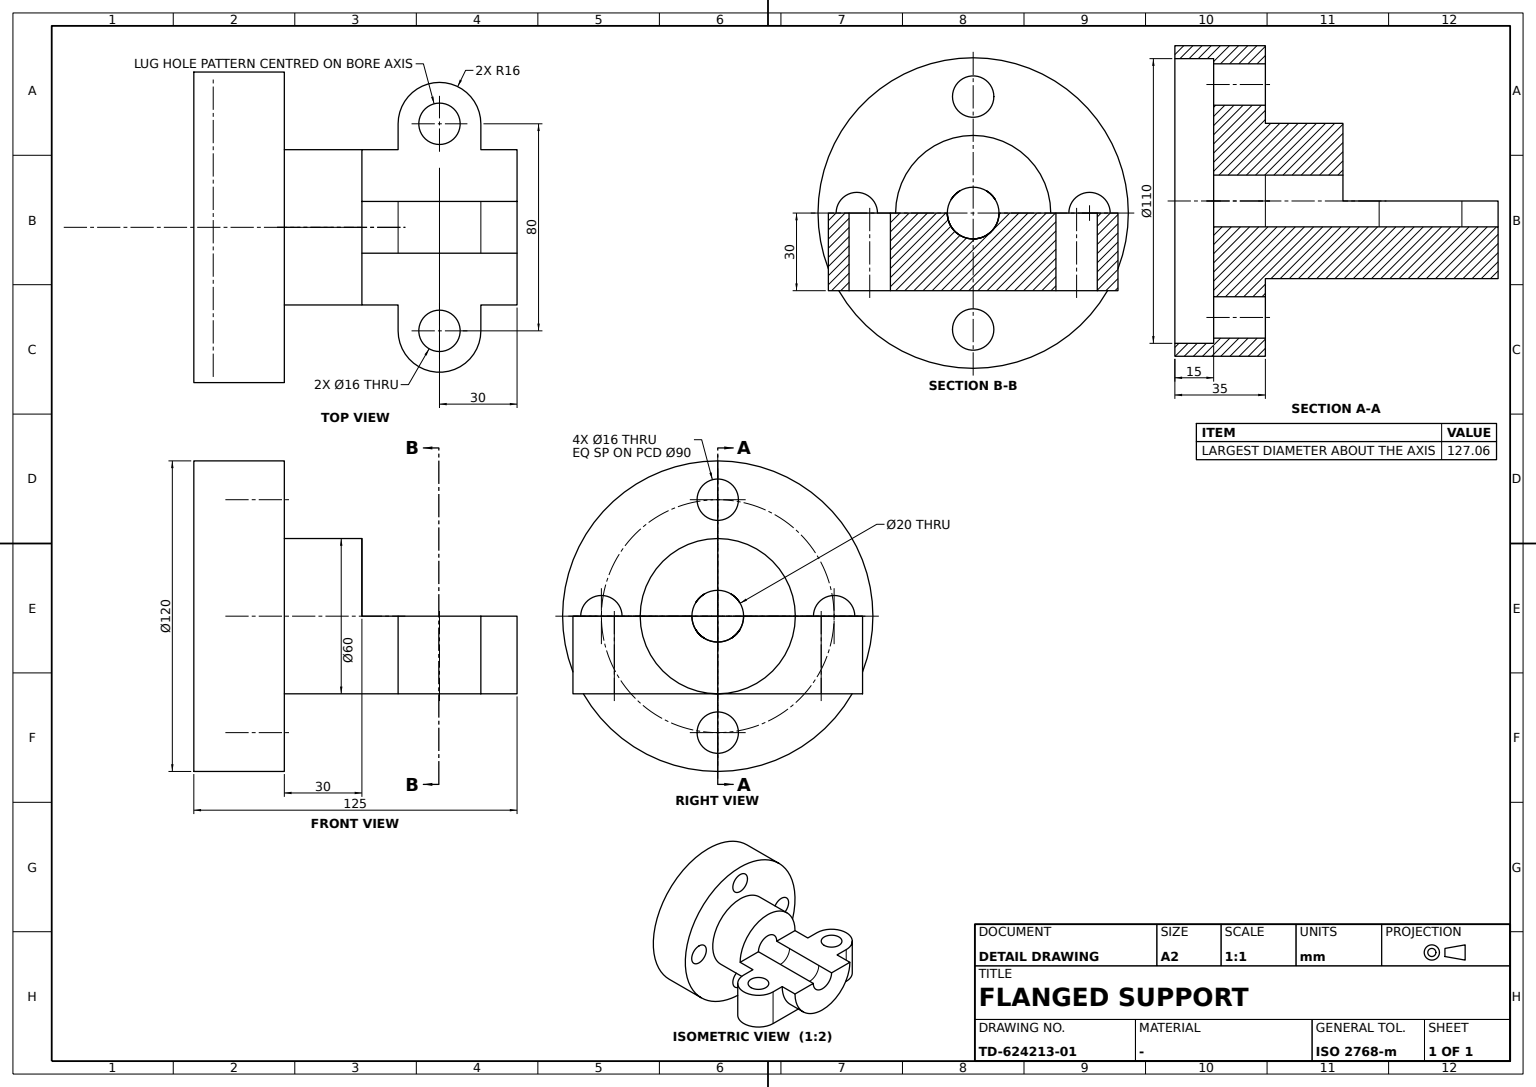
ISO-10303-21;
HEADER;
FILE_DESCRIPTION((''),'2;1');
FILE_NAME('','',(''),(''),'','','');
FILE_SCHEMA(('AUTOMOTIVE_DESIGN'));
ENDSEC;
DATA;
#1=APPLICATION_CONTEXT('');
#2=PRODUCT_CONTEXT('',#1,'mechanical');
#3=PRODUCT('','','',(#2));
#4=PRODUCT_DEFINITION_FORMATION('','',#3);
#5=PRODUCT_DEFINITION_CONTEXT('',#1,'design');
#6=PRODUCT_DEFINITION('','',#4,#5);
#7=PRODUCT_DEFINITION_SHAPE('','',#6);
#8=(LENGTH_UNIT()NAMED_UNIT(*)SI_UNIT(.MILLI.,.METRE.));
#9=(NAMED_UNIT(*)PLANE_ANGLE_UNIT()SI_UNIT($,.RADIAN.));
#10=(NAMED_UNIT(*)SI_UNIT($,.STERADIAN.)SOLID_ANGLE_UNIT());
#11=UNCERTAINTY_MEASURE_WITH_UNIT(LENGTH_MEASURE(1.E-05),#8,'distance_accuracy_value','');
#12=(GEOMETRIC_REPRESENTATION_CONTEXT(3)GLOBAL_UNCERTAINTY_ASSIGNED_CONTEXT((#11))GLOBAL_UNIT_ASSIGNED_CONTEXT((#8,#9,#10))REPRESENTATION_CONTEXT('',''));
#13=CARTESIAN_POINT('',(30.,0.,35.));
#14=VERTEX_POINT('',#13);
#15=CARTESIAN_POINT('',(-30.,0.,35.));
#16=VERTEX_POINT('',#15);
#17=CARTESIAN_POINT('',(0.,0.,35.));
#18=DIRECTION('',(0.,0.,1.));
#19=DIRECTION('',(1.,0.,0.));
#20=AXIS2_PLACEMENT_3D('',#17,#18,#19);
#21=CIRCLE('',#20,30.);
#22=EDGE_CURVE('',#14,#16,#21,.T.);
#23=ORIENTED_EDGE('',*,*,#22,.F.);
#24=EDGE_CURVE('',#16,#14,#21,.T.);
#25=ORIENTED_EDGE('',*,*,#24,.F.);
#26=EDGE_LOOP('',(#23,#25));
#27=FACE_BOUND('',#26,.T.);
#28=CARTESIAN_POINT('',(-8.,45.,35.));
#29=VERTEX_POINT('',#28);
#30=CARTESIAN_POINT('',(8.,45.,35.));
#31=VERTEX_POINT('',#30);
#32=CARTESIAN_POINT('',(0.,45.,35.));
#33=AXIS2_PLACEMENT_3D('',#32,#18,#19);
#34=CIRCLE('',#33,8.);
#35=EDGE_CURVE('',#29,#31,#34,.T.);
#36=ORIENTED_EDGE('',*,*,#35,.F.);
#37=EDGE_CURVE('',#31,#29,#34,.T.);
#38=ORIENTED_EDGE('',*,*,#37,.F.);
#39=EDGE_LOOP('',(#36,#38));
#40=FACE_BOUND('',#39,.T.);
#41=CARTESIAN_POINT('',(-45.,8.,35.));
#42=VERTEX_POINT('',#41);
#43=CARTESIAN_POINT('',(-45.,-8.,35.));
#44=VERTEX_POINT('',#43);
#45=CARTESIAN_POINT('',(-45.,0.,35.));
#46=DIRECTION('',(0.,1.,0.));
#47=AXIS2_PLACEMENT_3D('',#45,#18,#46);
#48=CIRCLE('',#47,8.);
#49=EDGE_CURVE('',#42,#44,#48,.T.);
#50=ORIENTED_EDGE('',*,*,#49,.F.);
#51=EDGE_CURVE('',#44,#42,#48,.T.);
#52=ORIENTED_EDGE('',*,*,#51,.F.);
#53=EDGE_LOOP('',(#50,#52));
#54=FACE_BOUND('',#53,.T.);
#55=CARTESIAN_POINT('',(45.,8.,35.));
#56=VERTEX_POINT('',#55);
#57=CARTESIAN_POINT('',(45.,-8.,35.));
#58=VERTEX_POINT('',#57);
#59=CARTESIAN_POINT('',(45.,0.,35.));
#60=DIRECTION('',(0.,-1.,0.));
#61=AXIS2_PLACEMENT_3D('',#59,#18,#60);
#62=CIRCLE('',#61,8.);
#63=EDGE_CURVE('',#56,#58,#62,.T.);
#64=ORIENTED_EDGE('',*,*,#63,.F.);
#65=EDGE_CURVE('',#58,#56,#62,.T.);
#66=ORIENTED_EDGE('',*,*,#65,.F.);
#67=EDGE_LOOP('',(#64,#66));
#68=FACE_BOUND('',#67,.T.);
#69=CARTESIAN_POINT('',(-8.,-45.,35.));
#70=VERTEX_POINT('',#69);
#71=CARTESIAN_POINT('',(8.,-45.,35.));
#72=VERTEX_POINT('',#71);
#73=CARTESIAN_POINT('',(0.,-45.,35.));
#74=DIRECTION('',(-1.,0.,0.));
#75=AXIS2_PLACEMENT_3D('',#73,#18,#74);
#76=CIRCLE('',#75,8.);
#77=EDGE_CURVE('',#70,#72,#76,.T.);
#78=ORIENTED_EDGE('',*,*,#77,.F.);
#79=EDGE_CURVE('',#72,#70,#76,.T.);
#80=ORIENTED_EDGE('',*,*,#79,.F.);
#81=EDGE_LOOP('',(#78,#80));
#82=FACE_BOUND('',#81,.T.);
#83=CARTESIAN_POINT('',(60.,0.,35.));
#84=VERTEX_POINT('',#83);
#85=CARTESIAN_POINT('',(-60.,0.,35.));
#86=VERTEX_POINT('',#85);
#87=CIRCLE('',#20,60.);
#88=EDGE_CURVE('',#84,#86,#87,.T.);
#89=ORIENTED_EDGE('',*,*,#88,.T.);
#90=EDGE_CURVE('',#86,#84,#87,.T.);
#91=ORIENTED_EDGE('',*,*,#90,.T.);
#92=EDGE_LOOP('',(#89,#91));
#93=FACE_OUTER_BOUND('',#92,.T.);
#94=PLANE('',#20);
#95=ADVANCED_FACE('',(#27,#40,#54,#68,#82,#93),#94,.T.);
#96=CARTESIAN_POINT('',(60.,0.,0.));
#97=VERTEX_POINT('',#96);
#98=CARTESIAN_POINT('',(60.,0.,17.5));
#99=VECTOR('',#18,1000.);
#100=LINE('',#98,#99);
#101=EDGE_CURVE('',#97,#84,#100,.T.);
#102=ORIENTED_EDGE('',*,*,#101,.F.);
#103=CARTESIAN_POINT('',(-60.,0.,0.));
#104=VERTEX_POINT('',#103);
#105=CARTESIAN_POINT('',(0.,0.,0.));
#106=AXIS2_PLACEMENT_3D('',#105,#18,#19);
#107=CIRCLE('',#106,60.);
#108=EDGE_CURVE('',#97,#104,#107,.T.);
#109=ORIENTED_EDGE('',*,*,#108,.T.);
#110=CARTESIAN_POINT('',(-60.,0.,17.5));
#111=LINE('',#110,#99);
#112=EDGE_CURVE('',#104,#86,#111,.T.);
#113=ORIENTED_EDGE('',*,*,#112,.T.);
#114=ORIENTED_EDGE('',*,*,#88,.F.);
#115=EDGE_LOOP('',(#102,#109,#113,#114));
#116=FACE_OUTER_BOUND('',#115,.T.);
#117=CARTESIAN_POINT('',(0.,0.,17.5));
#118=DIRECTION('',(0.,0.,-1.));
#119=AXIS2_PLACEMENT_3D('',#117,#118,#19);
#120=CYLINDRICAL_SURFACE('',#119,60.);
#121=ADVANCED_FACE('',(#116),#120,.T.);
#122=CARTESIAN_POINT('',(0.,30.,111.));
#123=VERTEX_POINT('',#122);
#124=CARTESIAN_POINT('',(30.,0.,111.));
#125=VERTEX_POINT('',#124);
#126=CARTESIAN_POINT('',(0.,0.,111.));
#127=AXIS2_PLACEMENT_3D('',#126,#118,#46);
#128=CIRCLE('',#127,30.);
#129=EDGE_CURVE('',#123,#125,#128,.T.);
#130=ORIENTED_EDGE('',*,*,#129,.T.);
#131=CARTESIAN_POINT('',(30.,40.,111.));
#132=VERTEX_POINT('',#131);
#133=CARTESIAN_POINT('',(30.,20.,111.));
#134=VECTOR('',#60,1000.);
#135=LINE('',#133,#134);
#136=EDGE_CURVE('',#132,#125,#135,.T.);
#137=ORIENTED_EDGE('',*,*,#136,.F.);
#138=CARTESIAN_POINT('',(0.,40.,111.));
#139=VERTEX_POINT('',#138);
#140=CARTESIAN_POINT('',(15.,40.,111.));
#141=VECTOR('',#19,1000.);
#142=LINE('',#140,#141);
#143=EDGE_CURVE('',#139,#132,#142,.T.);
#144=ORIENTED_EDGE('',*,*,#143,.F.);
#145=CARTESIAN_POINT('',(0.,35.,111.));
#146=LINE('',#145,#134);
#147=EDGE_CURVE('',#139,#123,#146,.T.);
#148=ORIENTED_EDGE('',*,*,#147,.T.);
#149=EDGE_LOOP('',(#130,#137,#144,#148));
#150=FACE_OUTER_BOUND('',#149,.T.);
#151=CARTESIAN_POINT('',(0.,-40.,111.));
#152=AXIS2_PLACEMENT_3D('',#151,#118,#46);
#153=PLANE('',#152);
#154=ADVANCED_FACE('',(#150),#153,.F.);
#155=CARTESIAN_POINT('',(0.,-48.,95.));
#156=VERTEX_POINT('',#155);
#157=CARTESIAN_POINT('',(30.,-48.,95.));
#158=VERTEX_POINT('',#157);
#159=CARTESIAN_POINT('',(15.,-48.,95.));
#160=LINE('',#159,#141);
#161=EDGE_CURVE('',#156,#158,#160,.T.);
#162=ORIENTED_EDGE('',*,*,#161,.T.);
#163=CARTESIAN_POINT('',(30.,-32.,95.));
#164=VERTEX_POINT('',#163);
#165=CARTESIAN_POINT('',(30.,-40.,95.));
#166=AXIS2_PLACEMENT_3D('',#165,#19,#46);
#167=CIRCLE('',#166,8.);
#168=EDGE_CURVE('',#158,#164,#167,.T.);
#169=ORIENTED_EDGE('',*,*,#168,.T.);
#170=CARTESIAN_POINT('',(0.,-32.,95.));
#171=VERTEX_POINT('',#170);
#172=CARTESIAN_POINT('',(15.,-32.,95.));
#173=LINE('',#172,#141);
#174=EDGE_CURVE('',#171,#164,#173,.T.);
#175=ORIENTED_EDGE('',*,*,#174,.F.);
#176=CARTESIAN_POINT('',(0.,-40.,95.));
#177=AXIS2_PLACEMENT_3D('',#176,#19,#46);
#178=CIRCLE('',#177,8.);
#179=EDGE_CURVE('',#156,#171,#178,.T.);
#180=ORIENTED_EDGE('',*,*,#179,.F.);
#181=EDGE_LOOP('',(#162,#169,#175,#180));
#182=FACE_OUTER_BOUND('',#181,.T.);
#183=CARTESIAN_POINT('',(15.,-40.,95.));
#184=AXIS2_PLACEMENT_3D('',#183,#74,#46);
#185=CYLINDRICAL_SURFACE('',#184,8.);
#186=ADVANCED_FACE('',(#182),#185,.F.);
#187=CARTESIAN_POINT('',(0.,32.,95.));
#188=VERTEX_POINT('',#187);
#189=CARTESIAN_POINT('',(0.,48.,95.));
#190=VERTEX_POINT('',#189);
#191=CARTESIAN_POINT('',(0.,40.,95.));
#192=AXIS2_PLACEMENT_3D('',#191,#19,#46);
#193=CIRCLE('',#192,8.);
#194=EDGE_CURVE('',#188,#190,#193,.T.);
#195=ORIENTED_EDGE('',*,*,#194,.F.);
#196=CARTESIAN_POINT('',(30.,32.,95.));
#197=VERTEX_POINT('',#196);
#198=CARTESIAN_POINT('',(15.,32.,95.));
#199=LINE('',#198,#141);
#200=EDGE_CURVE('',#188,#197,#199,.T.);
#201=ORIENTED_EDGE('',*,*,#200,.T.);
#202=CARTESIAN_POINT('',(30.,48.,95.));
#203=VERTEX_POINT('',#202);
#204=CARTESIAN_POINT('',(30.,40.,95.));
#205=AXIS2_PLACEMENT_3D('',#204,#19,#46);
#206=CIRCLE('',#205,8.);
#207=EDGE_CURVE('',#197,#203,#206,.T.);
#208=ORIENTED_EDGE('',*,*,#207,.T.);
#209=CARTESIAN_POINT('',(15.,48.,95.));
#210=LINE('',#209,#141);
#211=EDGE_CURVE('',#190,#203,#210,.T.);
#212=ORIENTED_EDGE('',*,*,#211,.F.);
#213=EDGE_LOOP('',(#195,#201,#208,#212));
#214=FACE_OUTER_BOUND('',#213,.T.);
#215=CARTESIAN_POINT('',(15.,40.,95.));
#216=AXIS2_PLACEMENT_3D('',#215,#74,#46);
#217=CYLINDRICAL_SURFACE('',#216,8.);
#218=ADVANCED_FACE('',(#214),#217,.F.);
#219=VERTEX_POINT('',#151);
#220=CARTESIAN_POINT('',(30.,-40.,111.));
#221=VERTEX_POINT('',#220);
#222=CARTESIAN_POINT('',(15.,-40.,111.));
#223=LINE('',#222,#141);
#224=EDGE_CURVE('',#219,#221,#223,.T.);
#225=ORIENTED_EDGE('',*,*,#224,.F.);
#226=CARTESIAN_POINT('',(0.,-40.,79.));
#227=VERTEX_POINT('',#226);
#228=CIRCLE('',#177,16.);
#229=EDGE_CURVE('',#219,#227,#228,.T.);
#230=ORIENTED_EDGE('',*,*,#229,.T.);
#231=CARTESIAN_POINT('',(30.,-40.,79.));
#232=VERTEX_POINT('',#231);
#233=CARTESIAN_POINT('',(15.,-40.,79.));
#234=LINE('',#233,#141);
#235=EDGE_CURVE('',#227,#232,#234,.T.);
#236=ORIENTED_EDGE('',*,*,#235,.T.);
#237=CIRCLE('',#166,16.);
#238=EDGE_CURVE('',#221,#232,#237,.T.);
#239=ORIENTED_EDGE('',*,*,#238,.F.);
#240=EDGE_LOOP('',(#225,#230,#236,#239));
#241=FACE_OUTER_BOUND('',#240,.T.);
#242=CYLINDRICAL_SURFACE('',#184,16.);
#243=ADVANCED_FACE('',(#241),#242,.T.);
#244=CARTESIAN_POINT('',(-10.,0.,65.));
#245=VERTEX_POINT('',#244);
#246=CARTESIAN_POINT('',(0.,-10.,65.));
#247=VERTEX_POINT('',#246);
#248=CARTESIAN_POINT('',(0.,0.,65.));
#249=AXIS2_PLACEMENT_3D('',#248,#18,#19);
#250=CIRCLE('',#249,10.);
#251=EDGE_CURVE('',#245,#247,#250,.T.);
#252=ORIENTED_EDGE('',*,*,#251,.T.);
#253=CARTESIAN_POINT('',(0.,-10.,79.));
#254=VERTEX_POINT('',#253);
#255=CARTESIAN_POINT('',(0.,-10.,72.));
#256=LINE('',#255,#99);
#257=EDGE_CURVE('',#247,#254,#256,.T.);
#258=ORIENTED_EDGE('',*,*,#257,.T.);
#259=CARTESIAN_POINT('',(10.,0.,79.));
#260=VERTEX_POINT('',#259);
#261=CARTESIAN_POINT('',(1.308997,-10.,79.));
#262=CARTESIAN_POINT('',(2.617479,-9.739727,79.));
#263=CARTESIAN_POINT('',(5.03619,-8.737864,79.));
#264=CARTESIAN_POINT('',(6.145467,-7.996668,79.));
#265=CARTESIAN_POINT('',(7.996668,-6.145467,79.));
#266=CARTESIAN_POINT('',(8.737864,-5.03619,79.));
#267=CARTESIAN_POINT('',(9.739727,-2.617479,79.));
#268=CARTESIAN_POINT('',(10.,-1.308997,79.));
#269=B_SPLINE_CURVE_WITH_KNOTS('',3,(#253,#261,#262,#263,#264,#265,#266,#267,#268,#259),.UNSPECIFIED.,.F.,.F.,(4,2,2,2,4),(0.,0.25,0.5,0.75,1.),.UNSPECIFIED.);
#270=EDGE_CURVE('',#254,#260,#269,.T.);
#271=ORIENTED_EDGE('',*,*,#270,.T.);
#272=CARTESIAN_POINT('',(10.,0.,35.));
#273=VERTEX_POINT('',#272);
#274=CARTESIAN_POINT('',(10.,0.,62.5));
#275=LINE('',#274,#99);
#276=EDGE_CURVE('',#273,#260,#275,.T.);
#277=ORIENTED_EDGE('',*,*,#276,.F.);
#278=CARTESIAN_POINT('',(0.,-10.,35.));
#279=VERTEX_POINT('',#278);
#280=CARTESIAN_POINT('',(3.141593,-10.,35.));
#281=CARTESIAN_POINT('',(6.286116,-8.76985,35.));
#282=CARTESIAN_POINT('',(8.76985,-6.286116,35.));
#283=CARTESIAN_POINT('',(10.,-3.141593,35.));
#284=B_SPLINE_CURVE_WITH_KNOTS('',5,(#278,#280,#281,#282,#283,#272),.UNSPECIFIED.,.F.,.F.,(6,6),(0.,1.),.UNSPECIFIED.);
#285=EDGE_CURVE('',#279,#273,#284,.T.);
#286=ORIENTED_EDGE('',*,*,#285,.F.);
#287=CARTESIAN_POINT('',(-10.,0.,35.));
#288=VERTEX_POINT('',#287);
#289=CARTESIAN_POINT('',(-10.,-3.141593,35.));
#290=CARTESIAN_POINT('',(-8.76985,-6.286116,35.));
#291=CARTESIAN_POINT('',(-6.286116,-8.76985,35.));
#292=CARTESIAN_POINT('',(-3.141593,-10.,35.));
#293=B_SPLINE_CURVE_WITH_KNOTS('',5,(#287,#289,#290,#291,#292,#278),.UNSPECIFIED.,.F.,.F.,(6,6),(0.,1.),.UNSPECIFIED.);
#294=EDGE_CURVE('',#288,#279,#293,.T.);
#295=ORIENTED_EDGE('',*,*,#294,.F.);
#296=CARTESIAN_POINT('',(-10.,0.,62.5));
#297=LINE('',#296,#99);
#298=EDGE_CURVE('',#288,#245,#297,.T.);
#299=ORIENTED_EDGE('',*,*,#298,.T.);
#300=EDGE_LOOP('',(#252,#258,#271,#277,#286,#295,#299));
#301=FACE_OUTER_BOUND('',#300,.T.);
#302=CARTESIAN_POINT('',(0.,0.,62.5));
#303=AXIS2_PLACEMENT_3D('',#302,#118,#19);
#304=CYLINDRICAL_SURFACE('',#303,10.);
#305=ADVANCED_FACE('',(#301),#304,.F.);
#306=CARTESIAN_POINT('',(-45.,8.,15.));
#307=VERTEX_POINT('',#306);
#308=CARTESIAN_POINT('',(-45.,8.,16.84));
#309=VECTOR('',#118,1000.);
#310=LINE('',#308,#309);
#311=EDGE_CURVE('',#42,#307,#310,.T.);
#312=ORIENTED_EDGE('',*,*,#311,.T.);
#313=CARTESIAN_POINT('',(-45.,-8.,15.));
#314=VERTEX_POINT('',#313);
#315=CARTESIAN_POINT('',(-45.,0.,15.));
#316=AXIS2_PLACEMENT_3D('',#315,#118,#19);
#317=CIRCLE('',#316,8.);
#318=EDGE_CURVE('',#307,#314,#317,.T.);
#319=ORIENTED_EDGE('',*,*,#318,.T.);
#320=CARTESIAN_POINT('',(-45.,-8.,16.84));
#321=LINE('',#320,#309);
#322=EDGE_CURVE('',#44,#314,#321,.T.);
#323=ORIENTED_EDGE('',*,*,#322,.F.);
#324=ORIENTED_EDGE('',*,*,#51,.T.);
#325=EDGE_LOOP('',(#312,#319,#323,#324));
#326=FACE_OUTER_BOUND('',#325,.T.);
#327=CARTESIAN_POINT('',(-45.,0.,16.84));
#328=AXIS2_PLACEMENT_3D('',#327,#118,#46);
#329=CYLINDRICAL_SURFACE('',#328,8.);
#330=ADVANCED_FACE('',(#326),#329,.F.);
#331=CARTESIAN_POINT('',(0.,-10.,125.));
#332=VERTEX_POINT('',#331);
#333=CARTESIAN_POINT('',(0.,-10.,111.));
#334=VERTEX_POINT('',#333);
#335=CARTESIAN_POINT('',(0.,-10.,118.));
#336=LINE('',#335,#309);
#337=EDGE_CURVE('',#332,#334,#336,.T.);
#338=ORIENTED_EDGE('',*,*,#337,.F.);
#339=CARTESIAN_POINT('',(10.,0.,125.));
#340=VERTEX_POINT('',#339);
#341=CARTESIAN_POINT('',(0.,0.,125.));
#342=AXIS2_PLACEMENT_3D('',#341,#18,#19);
#343=CIRCLE('',#342,10.);
#344=EDGE_CURVE('',#332,#340,#343,.T.);
#345=ORIENTED_EDGE('',*,*,#344,.T.);
#346=CARTESIAN_POINT('',(10.,0.,111.));
#347=VERTEX_POINT('',#346);
#348=EDGE_CURVE('',#347,#340,#275,.T.);
#349=ORIENTED_EDGE('',*,*,#348,.F.);
#350=CARTESIAN_POINT('',(3.141593,-10.,111.));
#351=CARTESIAN_POINT('',(6.286116,-8.76985,111.));
#352=CARTESIAN_POINT('',(8.76985,-6.286116,111.));
#353=CARTESIAN_POINT('',(10.,-3.141593,111.));
#354=B_SPLINE_CURVE_WITH_KNOTS('',5,(#333,#350,#351,#352,#353,#346),.UNSPECIFIED.,.F.,.F.,(6,6),(0.,1.),.UNSPECIFIED.);
#355=EDGE_CURVE('',#334,#347,#354,.T.);
#356=ORIENTED_EDGE('',*,*,#355,.F.);
#357=EDGE_LOOP('',(#338,#345,#349,#356));
#358=FACE_OUTER_BOUND('',#357,.T.);
#359=ADVANCED_FACE('',(#358),#304,.F.);
#360=CARTESIAN_POINT('',(0.,-30.,79.));
#361=VERTEX_POINT('',#360);
#362=CARTESIAN_POINT('',(0.,-30.,65.));
#363=VERTEX_POINT('',#362);
#364=CARTESIAN_POINT('',(0.,-30.,62.5));
#365=LINE('',#364,#309);
#366=EDGE_CURVE('',#361,#363,#365,.T.);
#367=ORIENTED_EDGE('',*,*,#366,.T.);
#368=CARTESIAN_POINT('',(-30.,0.,65.));
#369=VERTEX_POINT('',#368);
#370=CIRCLE('',#249,30.);
#371=EDGE_CURVE('',#369,#363,#370,.T.);
#372=ORIENTED_EDGE('',*,*,#371,.F.);
#373=CARTESIAN_POINT('',(-30.,0.,62.5));
#374=LINE('',#373,#99);
#375=EDGE_CURVE('',#16,#369,#374,.T.);
#376=ORIENTED_EDGE('',*,*,#375,.F.);
#377=ORIENTED_EDGE('',*,*,#24,.T.);
#378=CARTESIAN_POINT('',(30.,0.,79.));
#379=VERTEX_POINT('',#378);
#380=CARTESIAN_POINT('',(30.,0.,62.5));
#381=LINE('',#380,#99);
#382=EDGE_CURVE('',#14,#379,#381,.T.);
#383=ORIENTED_EDGE('',*,*,#382,.T.);
#384=CARTESIAN_POINT('',(0.,0.,79.));
#385=AXIS2_PLACEMENT_3D('',#384,#18,#60);
#386=CIRCLE('',#385,30.);
#387=EDGE_CURVE('',#361,#379,#386,.T.);
#388=ORIENTED_EDGE('',*,*,#387,.F.);
#389=EDGE_LOOP('',(#367,#372,#376,#377,#383,#388));
#390=FACE_OUTER_BOUND('',#389,.T.);
#391=CYLINDRICAL_SURFACE('',#303,30.);
#392=ADVANCED_FACE('',(#390),#391,.T.);
#393=ORIENTED_EDGE('',*,*,#194,.T.);
#394=EDGE_CURVE('',#190,#188,#193,.T.);
#395=ORIENTED_EDGE('',*,*,#394,.T.);
#396=EDGE_LOOP('',(#393,#395));
#397=FACE_BOUND('',#396,.T.);
#398=CARTESIAN_POINT('',(0.,10.,125.));
#399=VERTEX_POINT('',#398);
#400=CARTESIAN_POINT('',(0.,30.,125.));
#401=VERTEX_POINT('',#400);
#402=CARTESIAN_POINT('',(0.,20.,125.));
#403=VECTOR('',#46,1000.);
#404=LINE('',#402,#403);
#405=EDGE_CURVE('',#399,#401,#404,.T.);
#406=ORIENTED_EDGE('',*,*,#405,.T.);
#407=CARTESIAN_POINT('',(0.,30.,62.5));
#408=LINE('',#407,#309);
#409=EDGE_CURVE('',#401,#123,#408,.T.);
#410=ORIENTED_EDGE('',*,*,#409,.T.);
#411=ORIENTED_EDGE('',*,*,#147,.F.);
#412=CARTESIAN_POINT('',(0.,56.,95.));
#413=VERTEX_POINT('',#412);
#414=CIRCLE('',#192,16.);
#415=EDGE_CURVE('',#413,#139,#414,.T.);
#416=ORIENTED_EDGE('',*,*,#415,.F.);
#417=CARTESIAN_POINT('',(0.,40.,79.));
#418=VERTEX_POINT('',#417);
#419=EDGE_CURVE('',#418,#413,#414,.T.);
#420=ORIENTED_EDGE('',*,*,#419,.F.);
#421=CARTESIAN_POINT('',(0.,30.,79.));
#422=VERTEX_POINT('',#421);
#423=CARTESIAN_POINT('',(0.,35.,79.));
#424=LINE('',#423,#403);
#425=EDGE_CURVE('',#422,#418,#424,.T.);
#426=ORIENTED_EDGE('',*,*,#425,.F.);
#427=CARTESIAN_POINT('',(0.,30.,65.));
#428=VERTEX_POINT('',#427);
#429=EDGE_CURVE('',#422,#428,#408,.T.);
#430=ORIENTED_EDGE('',*,*,#429,.T.);
#431=CARTESIAN_POINT('',(0.,10.,65.));
#432=VERTEX_POINT('',#431);
#433=CARTESIAN_POINT('',(0.,20.,65.));
#434=LINE('',#433,#403);
#435=EDGE_CURVE('',#432,#428,#434,.T.);
#436=ORIENTED_EDGE('',*,*,#435,.F.);
#437=CARTESIAN_POINT('',(0.,10.,79.));
#438=VERTEX_POINT('',#437);
#439=CARTESIAN_POINT('',(0.,10.,72.));
#440=LINE('',#439,#99);
#441=EDGE_CURVE('',#432,#438,#440,.T.);
#442=ORIENTED_EDGE('',*,*,#441,.T.);
#443=CARTESIAN_POINT('',(0.,10.,111.));
#444=VERTEX_POINT('',#443);
#445=CARTESIAN_POINT('',(0.,10.,95.));
#446=LINE('',#445,#309);
#447=EDGE_CURVE('',#444,#438,#446,.T.);
#448=ORIENTED_EDGE('',*,*,#447,.F.);
#449=CARTESIAN_POINT('',(0.,10.,118.));
#450=LINE('',#449,#99);
#451=EDGE_CURVE('',#444,#399,#450,.T.);
#452=ORIENTED_EDGE('',*,*,#451,.T.);
#453=EDGE_LOOP('',(#406,#410,#411,#416,#420,#426,#430,#436,#442,#448,#452));
#454=FACE_OUTER_BOUND('',#453,.T.);
#455=AXIS2_PLACEMENT_3D('',#105,#19,#46);
#456=PLANE('',#455);
#457=ADVANCED_FACE('',(#397,#454),#456,.F.);
#458=EDGE_CURVE('',#379,#422,#386,.T.);
#459=ORIENTED_EDGE('',*,*,#458,.T.);
#460=ORIENTED_EDGE('',*,*,#425,.T.);
#461=CARTESIAN_POINT('',(30.,40.,79.));
#462=VERTEX_POINT('',#461);
#463=CARTESIAN_POINT('',(15.,40.,79.));
#464=LINE('',#463,#141);
#465=EDGE_CURVE('',#418,#462,#464,.T.);
#466=ORIENTED_EDGE('',*,*,#465,.T.);
#467=CARTESIAN_POINT('',(30.,20.,79.));
#468=LINE('',#467,#403);
#469=EDGE_CURVE('',#379,#462,#468,.T.);
#470=ORIENTED_EDGE('',*,*,#469,.F.);
#471=EDGE_LOOP('',(#459,#460,#466,#470));
#472=FACE_OUTER_BOUND('',#471,.T.);
#473=AXIS2_PLACEMENT_3D('',#417,#18,#60);
#474=PLANE('',#473);
#475=ADVANCED_FACE('',(#472),#474,.F.);
#476=CARTESIAN_POINT('',(0.,-30.,111.));
#477=VERTEX_POINT('',#476);
#478=EDGE_CURVE('',#125,#477,#128,.T.);
#479=ORIENTED_EDGE('',*,*,#478,.F.);
#480=CARTESIAN_POINT('',(30.,0.,125.));
#481=VERTEX_POINT('',#480);
#482=EDGE_CURVE('',#125,#481,#381,.T.);
#483=ORIENTED_EDGE('',*,*,#482,.T.);
#484=CARTESIAN_POINT('',(0.,-30.,125.));
#485=VERTEX_POINT('',#484);
#486=CIRCLE('',#342,30.);
#487=EDGE_CURVE('',#485,#481,#486,.T.);
#488=ORIENTED_EDGE('',*,*,#487,.F.);
#489=EDGE_CURVE('',#485,#477,#365,.T.);
#490=ORIENTED_EDGE('',*,*,#489,.T.);
#491=EDGE_LOOP('',(#479,#483,#488,#490));
#492=FACE_OUTER_BOUND('',#491,.T.);
#493=ADVANCED_FACE('',(#492),#391,.T.);
#494=EDGE_CURVE('',#314,#307,#317,.T.);
#495=ORIENTED_EDGE('',*,*,#494,.T.);
#496=ORIENTED_EDGE('',*,*,#311,.F.);
#497=ORIENTED_EDGE('',*,*,#49,.T.);
#498=ORIENTED_EDGE('',*,*,#322,.T.);
#499=EDGE_LOOP('',(#495,#496,#497,#498));
#500=FACE_OUTER_BOUND('',#499,.T.);
#501=ADVANCED_FACE('',(#500),#329,.F.);
#502=CARTESIAN_POINT('',(10.,3.141593,111.));
#503=CARTESIAN_POINT('',(8.76985,6.286116,111.));
#504=CARTESIAN_POINT('',(6.286116,8.76985,111.));
#505=CARTESIAN_POINT('',(3.141593,10.,111.));
#506=B_SPLINE_CURVE_WITH_KNOTS('',5,(#346,#502,#503,#504,#505,#443),.UNSPECIFIED.,.F.,.F.,(6,6),(0.,1.),.UNSPECIFIED.);
#507=EDGE_CURVE('',#347,#444,#506,.T.);
#508=ORIENTED_EDGE('',*,*,#507,.F.);
#509=ORIENTED_EDGE('',*,*,#348,.T.);
#510=EDGE_CURVE('',#340,#399,#343,.T.);
#511=ORIENTED_EDGE('',*,*,#510,.T.);
#512=ORIENTED_EDGE('',*,*,#451,.F.);
#513=EDGE_LOOP('',(#508,#509,#511,#512));
#514=FACE_OUTER_BOUND('',#513,.T.);
#515=ADVANCED_FACE('',(#514),#304,.F.);
#516=ORIENTED_EDGE('',*,*,#344,.F.);
#517=CARTESIAN_POINT('',(0.,-20.,125.));
#518=LINE('',#517,#403);
#519=EDGE_CURVE('',#485,#332,#518,.T.);
#520=ORIENTED_EDGE('',*,*,#519,.F.);
#521=ORIENTED_EDGE('',*,*,#487,.T.);
#522=EDGE_CURVE('',#481,#401,#486,.T.);
#523=ORIENTED_EDGE('',*,*,#522,.T.);
#524=ORIENTED_EDGE('',*,*,#405,.F.);
#525=ORIENTED_EDGE('',*,*,#510,.F.);
#526=EDGE_LOOP('',(#516,#520,#521,#523,#524,#525));
#527=FACE_OUTER_BOUND('',#526,.T.);
#528=PLANE('',#342);
#529=ADVANCED_FACE('',(#527),#528,.T.);
#530=ORIENTED_EDGE('',*,*,#387,.T.);
#531=CARTESIAN_POINT('',(30.,-20.,79.));
#532=LINE('',#531,#403);
#533=EDGE_CURVE('',#232,#379,#532,.T.);
#534=ORIENTED_EDGE('',*,*,#533,.F.);
#535=ORIENTED_EDGE('',*,*,#235,.F.);
#536=CARTESIAN_POINT('',(0.,-35.,79.));
#537=LINE('',#536,#403);
#538=EDGE_CURVE('',#227,#361,#537,.T.);
#539=ORIENTED_EDGE('',*,*,#538,.T.);
#540=EDGE_LOOP('',(#530,#534,#535,#539));
#541=FACE_OUTER_BOUND('',#540,.T.);
#542=ADVANCED_FACE('',(#541),#474,.F.);
#543=ORIENTED_EDGE('',*,*,#112,.F.);
#544=EDGE_CURVE('',#104,#97,#107,.T.);
#545=ORIENTED_EDGE('',*,*,#544,.T.);
#546=ORIENTED_EDGE('',*,*,#101,.T.);
#547=ORIENTED_EDGE('',*,*,#90,.F.);
#548=EDGE_LOOP('',(#543,#545,#546,#547));
#549=FACE_OUTER_BOUND('',#548,.T.);
#550=ADVANCED_FACE('',(#549),#120,.T.);
#551=CARTESIAN_POINT('',(45.,8.,15.));
#552=VERTEX_POINT('',#551);
#553=CARTESIAN_POINT('',(45.,8.,16.84));
#554=LINE('',#553,#309);
#555=EDGE_CURVE('',#56,#552,#554,.T.);
#556=ORIENTED_EDGE('',*,*,#555,.T.);
#557=CARTESIAN_POINT('',(45.,-8.,15.));
#558=VERTEX_POINT('',#557);
#559=CARTESIAN_POINT('',(45.,0.,15.));
#560=AXIS2_PLACEMENT_3D('',#559,#118,#19);
#561=CIRCLE('',#560,8.);
#562=EDGE_CURVE('',#552,#558,#561,.T.);
#563=ORIENTED_EDGE('',*,*,#562,.T.);
#564=CARTESIAN_POINT('',(45.,-8.,16.84));
#565=LINE('',#564,#309);
#566=EDGE_CURVE('',#58,#558,#565,.T.);
#567=ORIENTED_EDGE('',*,*,#566,.F.);
#568=ORIENTED_EDGE('',*,*,#65,.T.);
#569=EDGE_LOOP('',(#556,#563,#567,#568));
#570=FACE_OUTER_BOUND('',#569,.T.);
#571=CARTESIAN_POINT('',(45.,0.,16.84));
#572=AXIS2_PLACEMENT_3D('',#571,#118,#60);
#573=CYLINDRICAL_SURFACE('',#572,8.);
#574=ADVANCED_FACE('',(#570),#573,.F.);
#575=CARTESIAN_POINT('',(10.,0.,15.));
#576=VERTEX_POINT('',#575);
#577=CARTESIAN_POINT('',(10.,0.,54.84));
#578=LINE('',#577,#309);
#579=EDGE_CURVE('',#273,#576,#578,.T.);
#580=ORIENTED_EDGE('',*,*,#579,.F.);
#581=CARTESIAN_POINT('',(0.,10.,35.));
#582=VERTEX_POINT('',#581);
#583=CARTESIAN_POINT('',(10.,3.141593,35.));
#584=CARTESIAN_POINT('',(8.76985,6.286116,35.));
#585=CARTESIAN_POINT('',(6.286116,8.76985,35.));
#586=CARTESIAN_POINT('',(3.141593,10.,35.));
#587=B_SPLINE_CURVE_WITH_KNOTS('',5,(#272,#583,#584,#585,#586,#581),.UNSPECIFIED.,.F.,.F.,(6,6),(0.,1.),.UNSPECIFIED.);
#588=EDGE_CURVE('',#273,#582,#587,.T.);
#589=ORIENTED_EDGE('',*,*,#588,.T.);
#590=CARTESIAN_POINT('',(0.,10.,15.));
#591=VERTEX_POINT('',#590);
#592=CARTESIAN_POINT('',(0.,10.,16.84));
#593=LINE('',#592,#309);
#594=EDGE_CURVE('',#582,#591,#593,.T.);
#595=ORIENTED_EDGE('',*,*,#594,.T.);
#596=CARTESIAN_POINT('',(1.035475,10.,15.));
#597=CARTESIAN_POINT('',(2.071108,9.86636,15.));
#598=CARTESIAN_POINT('',(3.083528,9.598273,15.));
#599=CARTESIAN_POINT('',(5.01583,8.805806,15.));
#600=CARTESIAN_POINT('',(6.682628,7.547344,15.));
#601=CARTESIAN_POINT('',(7.429877,6.812965,15.));
#602=CARTESIAN_POINT('',(8.738766,5.140658,15.));
#603=CARTESIAN_POINT('',(9.570775,3.185553,15.));
#604=CARTESIAN_POINT('',(9.857224,2.140738,15.));
#605=CARTESIAN_POINT('',(10.,1.070284,15.));
#606=B_SPLINE_CURVE_WITH_KNOTS('',5,(#590,#596,#597,#598,#599,#600,#601,#602,#603,#604,#605,#575),.UNSPECIFIED.,.F.,.F.,(6,3,3,6),(0.,7.321912465,14.646095776,22.214147767),.UNSPECIFIED.);
#607=EDGE_CURVE('',#591,#576,#606,.T.);
#608=ORIENTED_EDGE('',*,*,#607,.T.);
#609=EDGE_LOOP('',(#580,#589,#595,#608));
#610=FACE_OUTER_BOUND('',#609,.T.);
#611=CARTESIAN_POINT('',(3.141593,10.,15.));
#612=CARTESIAN_POINT('',(6.286116,8.76985,15.));
#613=CARTESIAN_POINT('',(8.76985,6.286116,15.));
#614=CARTESIAN_POINT('',(10.,3.141593,15.));
#615=B_SPLINE_SURFACE_WITH_KNOTS('',5,1,((#581,#590),(#586,#611),(#585,#612),(#584,#613),(#583,#614),(#272,#575)),.UNSPECIFIED.,.F.,.F.,.F.,(6,6),(2,2),(35.707963268,51.415926536),(76.,96.),.UNSPECIFIED.);
#616=ADVANCED_FACE('',(#610),#615,.F.);
#617=CARTESIAN_POINT('',(8.,45.,15.));
#618=VERTEX_POINT('',#617);
#619=CARTESIAN_POINT('',(8.,45.,16.84));
#620=LINE('',#619,#309);
#621=EDGE_CURVE('',#31,#618,#620,.T.);
#622=ORIENTED_EDGE('',*,*,#621,.F.);
#623=ORIENTED_EDGE('',*,*,#37,.T.);
#624=CARTESIAN_POINT('',(-8.,45.,15.));
#625=VERTEX_POINT('',#624);
#626=CARTESIAN_POINT('',(-8.,45.,16.84));
#627=LINE('',#626,#309);
#628=EDGE_CURVE('',#29,#625,#627,.T.);
#629=ORIENTED_EDGE('',*,*,#628,.T.);
#630=CARTESIAN_POINT('',(0.,45.,15.));
#631=AXIS2_PLACEMENT_3D('',#630,#118,#19);
#632=CIRCLE('',#631,8.);
#633=EDGE_CURVE('',#625,#618,#632,.T.);
#634=ORIENTED_EDGE('',*,*,#633,.T.);
#635=EDGE_LOOP('',(#622,#623,#629,#634));
#636=FACE_OUTER_BOUND('',#635,.T.);
#637=CARTESIAN_POINT('',(0.,45.,16.84));
#638=AXIS2_PLACEMENT_3D('',#637,#118,#19);
#639=CYLINDRICAL_SURFACE('',#638,8.);
#640=ADVANCED_FACE('',(#636),#639,.F.);
#641=CARTESIAN_POINT('',(8.,-45.,15.));
#642=VERTEX_POINT('',#641);
#643=CARTESIAN_POINT('',(-8.,-45.,15.));
#644=VERTEX_POINT('',#643);
#645=CARTESIAN_POINT('',(0.,-45.,15.));
#646=AXIS2_PLACEMENT_3D('',#645,#118,#19);
#647=CIRCLE('',#646,8.);
#648=EDGE_CURVE('',#642,#644,#647,.T.);
#649=ORIENTED_EDGE('',*,*,#648,.T.);
#650=CARTESIAN_POINT('',(-8.,-45.,16.84));
#651=LINE('',#650,#309);
#652=EDGE_CURVE('',#70,#644,#651,.T.);
#653=ORIENTED_EDGE('',*,*,#652,.F.);
#654=ORIENTED_EDGE('',*,*,#77,.T.);
#655=CARTESIAN_POINT('',(8.,-45.,16.84));
#656=LINE('',#655,#309);
#657=EDGE_CURVE('',#72,#642,#656,.T.);
#658=ORIENTED_EDGE('',*,*,#657,.T.);
#659=EDGE_LOOP('',(#649,#653,#654,#658));
#660=FACE_OUTER_BOUND('',#659,.T.);
#661=CARTESIAN_POINT('',(0.,-45.,16.84));
#662=AXIS2_PLACEMENT_3D('',#661,#118,#74);
#663=CYLINDRICAL_SURFACE('',#662,8.);
#664=ADVANCED_FACE('',(#660),#663,.F.);
#665=CARTESIAN_POINT('',(55.,0.,0.));
#666=VERTEX_POINT('',#665);
#667=CARTESIAN_POINT('',(-55.,0.,0.));
#668=VERTEX_POINT('',#667);
#669=AXIS2_PLACEMENT_3D('',#105,#118,#19);
#670=CIRCLE('',#669,55.);
#671=EDGE_CURVE('',#666,#668,#670,.T.);
#672=ORIENTED_EDGE('',*,*,#671,.T.);
#673=CARTESIAN_POINT('',(-55.,0.,15.));
#674=VERTEX_POINT('',#673);
#675=CARTESIAN_POINT('',(-55.,0.,7.5));
#676=LINE('',#675,#99);
#677=EDGE_CURVE('',#668,#674,#676,.T.);
#678=ORIENTED_EDGE('',*,*,#677,.T.);
#679=CARTESIAN_POINT('',(55.,0.,15.));
#680=VERTEX_POINT('',#679);
#681=CARTESIAN_POINT('',(0.,0.,15.));
#682=AXIS2_PLACEMENT_3D('',#681,#118,#19);
#683=CIRCLE('',#682,55.);
#684=EDGE_CURVE('',#680,#674,#683,.T.);
#685=ORIENTED_EDGE('',*,*,#684,.F.);
#686=CARTESIAN_POINT('',(55.,0.,7.5));
#687=LINE('',#686,#99);
#688=EDGE_CURVE('',#666,#680,#687,.T.);
#689=ORIENTED_EDGE('',*,*,#688,.F.);
#690=EDGE_LOOP('',(#672,#678,#685,#689));
#691=FACE_OUTER_BOUND('',#690,.T.);
#692=CARTESIAN_POINT('',(0.,0.,7.5));
#693=AXIS2_PLACEMENT_3D('',#692,#18,#19);
#694=CYLINDRICAL_SURFACE('',#693,55.);
#695=ADVANCED_FACE('',(#691),#694,.F.);
#696=EDGE_CURVE('',#674,#680,#683,.T.);
#697=ORIENTED_EDGE('',*,*,#696,.F.);
#698=ORIENTED_EDGE('',*,*,#677,.F.);
#699=EDGE_CURVE('',#668,#666,#670,.T.);
#700=ORIENTED_EDGE('',*,*,#699,.T.);
#701=ORIENTED_EDGE('',*,*,#688,.T.);
#702=EDGE_LOOP('',(#697,#698,#700,#701));
#703=FACE_OUTER_BOUND('',#702,.T.);
#704=ADVANCED_FACE('',(#703),#694,.F.);
#705=CARTESIAN_POINT('',(30.,56.,95.));
#706=VERTEX_POINT('',#705);
#707=CIRCLE('',#205,16.);
#708=EDGE_CURVE('',#462,#706,#707,.T.);
#709=ORIENTED_EDGE('',*,*,#708,.F.);
#710=ORIENTED_EDGE('',*,*,#465,.F.);
#711=ORIENTED_EDGE('',*,*,#419,.T.);
#712=CARTESIAN_POINT('',(15.,56.,95.));
#713=VECTOR('',#74,1000.);
#714=LINE('',#712,#713);
#715=EDGE_CURVE('',#706,#413,#714,.T.);
#716=ORIENTED_EDGE('',*,*,#715,.F.);
#717=EDGE_LOOP('',(#709,#710,#711,#716));
#718=FACE_OUTER_BOUND('',#717,.T.);
#719=CYLINDRICAL_SURFACE('',#216,16.);
#720=ADVANCED_FACE('',(#718),#719,.T.);
#721=ORIENTED_EDGE('',*,*,#161,.F.);
#722=EDGE_CURVE('',#171,#156,#178,.T.);
#723=ORIENTED_EDGE('',*,*,#722,.F.);
#724=ORIENTED_EDGE('',*,*,#174,.T.);
#725=EDGE_CURVE('',#164,#158,#167,.T.);
#726=ORIENTED_EDGE('',*,*,#725,.T.);
#727=EDGE_LOOP('',(#721,#723,#724,#726));
#728=FACE_OUTER_BOUND('',#727,.T.);
#729=ADVANCED_FACE('',(#728),#185,.F.);
#730=ORIENTED_EDGE('',*,*,#371,.T.);
#731=CARTESIAN_POINT('',(0.,-20.,65.));
#732=LINE('',#731,#403);
#733=EDGE_CURVE('',#363,#247,#732,.T.);
#734=ORIENTED_EDGE('',*,*,#733,.T.);
#735=ORIENTED_EDGE('',*,*,#251,.F.);
#736=EDGE_CURVE('',#432,#245,#250,.T.);
#737=ORIENTED_EDGE('',*,*,#736,.F.);
#738=ORIENTED_EDGE('',*,*,#435,.T.);
#739=EDGE_CURVE('',#428,#369,#370,.T.);
#740=ORIENTED_EDGE('',*,*,#739,.T.);
#741=EDGE_LOOP('',(#730,#734,#735,#737,#738,#740));
#742=FACE_OUTER_BOUND('',#741,.T.);
#743=CARTESIAN_POINT('',(-61.410713,0.,65.));
#744=AXIS2_PLACEMENT_3D('',#743,#18,#19);
#745=PLANE('',#744);
#746=ADVANCED_FACE('',(#742),#745,.T.);
#747=ORIENTED_EDGE('',*,*,#375,.T.);
#748=ORIENTED_EDGE('',*,*,#739,.F.);
#749=ORIENTED_EDGE('',*,*,#429,.F.);
#750=ORIENTED_EDGE('',*,*,#458,.F.);
#751=ORIENTED_EDGE('',*,*,#382,.F.);
#752=ORIENTED_EDGE('',*,*,#22,.T.);
#753=EDGE_LOOP('',(#747,#748,#749,#750,#751,#752));
#754=FACE_OUTER_BOUND('',#753,.T.);
#755=ADVANCED_FACE('',(#754),#391,.T.);
#756=CARTESIAN_POINT('',(0.,-10.,95.));
#757=LINE('',#756,#309);
#758=EDGE_CURVE('',#334,#254,#757,.T.);
#759=ORIENTED_EDGE('',*,*,#758,.T.);
#760=ORIENTED_EDGE('',*,*,#257,.F.);
#761=ORIENTED_EDGE('',*,*,#733,.F.);
#762=ORIENTED_EDGE('',*,*,#366,.F.);
#763=ORIENTED_EDGE('',*,*,#538,.F.);
#764=ORIENTED_EDGE('',*,*,#229,.F.);
#765=CARTESIAN_POINT('',(0.,-35.,111.));
#766=LINE('',#765,#134);
#767=EDGE_CURVE('',#477,#219,#766,.T.);
#768=ORIENTED_EDGE('',*,*,#767,.F.);
#769=ORIENTED_EDGE('',*,*,#489,.F.);
#770=ORIENTED_EDGE('',*,*,#519,.T.);
#771=ORIENTED_EDGE('',*,*,#337,.T.);
#772=EDGE_LOOP('',(#759,#760,#761,#762,#763,#764,#768,#769,#770,#771));
#773=FACE_OUTER_BOUND('',#772,.T.);
#774=ORIENTED_EDGE('',*,*,#722,.T.);
#775=ORIENTED_EDGE('',*,*,#179,.T.);
#776=EDGE_LOOP('',(#774,#775));
#777=FACE_BOUND('',#776,.T.);
#778=ADVANCED_FACE('',(#773,#777),#456,.F.);
#779=ORIENTED_EDGE('',*,*,#736,.T.);
#780=ORIENTED_EDGE('',*,*,#298,.F.);
#781=CARTESIAN_POINT('',(-3.141593,10.,35.));
#782=CARTESIAN_POINT('',(-6.286116,8.76985,35.));
#783=CARTESIAN_POINT('',(-8.76985,6.286116,35.));
#784=CARTESIAN_POINT('',(-10.,3.141593,35.));
#785=B_SPLINE_CURVE_WITH_KNOTS('',5,(#581,#781,#782,#783,#784,#287),.UNSPECIFIED.,.F.,.F.,(6,6),(0.,1.),.UNSPECIFIED.);
#786=EDGE_CURVE('',#582,#288,#785,.T.);
#787=ORIENTED_EDGE('',*,*,#786,.F.);
#788=ORIENTED_EDGE('',*,*,#588,.F.);
#789=ORIENTED_EDGE('',*,*,#276,.T.);
#790=CARTESIAN_POINT('',(10.,1.308997,79.));
#791=CARTESIAN_POINT('',(9.739727,2.617479,79.));
#792=CARTESIAN_POINT('',(8.737864,5.03619,79.));
#793=CARTESIAN_POINT('',(7.996668,6.145467,79.));
#794=CARTESIAN_POINT('',(6.145467,7.996668,79.));
#795=CARTESIAN_POINT('',(5.03619,8.737864,79.));
#796=CARTESIAN_POINT('',(2.617479,9.739727,79.));
#797=CARTESIAN_POINT('',(1.308997,10.,79.));
#798=B_SPLINE_CURVE_WITH_KNOTS('',3,(#259,#790,#791,#792,#793,#794,#795,#796,#797,#437),.UNSPECIFIED.,.F.,.F.,(4,2,2,2,4),(0.,0.25,0.5,0.75,1.),.UNSPECIFIED.);
#799=EDGE_CURVE('',#260,#438,#798,.T.);
#800=ORIENTED_EDGE('',*,*,#799,.T.);
#801=ORIENTED_EDGE('',*,*,#441,.F.);
#802=EDGE_LOOP('',(#779,#780,#787,#788,#789,#800,#801));
#803=FACE_OUTER_BOUND('',#802,.T.);
#804=ADVANCED_FACE('',(#803),#304,.F.);
#805=ORIENTED_EDGE('',*,*,#224,.T.);
#806=CARTESIAN_POINT('',(30.,-20.,111.));
#807=LINE('',#806,#134);
#808=EDGE_CURVE('',#125,#221,#807,.T.);
#809=ORIENTED_EDGE('',*,*,#808,.F.);
#810=ORIENTED_EDGE('',*,*,#478,.T.);
#811=ORIENTED_EDGE('',*,*,#767,.T.);
#812=EDGE_LOOP('',(#805,#809,#810,#811));
#813=FACE_OUTER_BOUND('',#812,.T.);
#814=ADVANCED_FACE('',(#813),#153,.F.);
#815=ORIENTED_EDGE('',*,*,#544,.F.);
#816=ORIENTED_EDGE('',*,*,#108,.F.);
#817=EDGE_LOOP('',(#815,#816));
#818=FACE_OUTER_BOUND('',#817,.T.);
#819=ORIENTED_EDGE('',*,*,#699,.F.);
#820=ORIENTED_EDGE('',*,*,#671,.F.);
#821=EDGE_LOOP('',(#819,#820));
#822=FACE_BOUND('',#821,.T.);
#823=PLANE('',#106);
#824=ADVANCED_FACE('',(#818,#822),#823,.F.);
#825=ORIENTED_EDGE('',*,*,#285,.T.);
#826=ORIENTED_EDGE('',*,*,#579,.T.);
#827=CARTESIAN_POINT('',(0.,-10.,15.));
#828=VERTEX_POINT('',#827);
#829=CARTESIAN_POINT('',(10.,-1.035475,15.));
#830=CARTESIAN_POINT('',(9.86636,-2.071108,15.));
#831=CARTESIAN_POINT('',(9.598273,-3.083528,15.));
#832=CARTESIAN_POINT('',(8.805806,-5.01583,15.));
#833=CARTESIAN_POINT('',(7.547344,-6.682628,15.));
#834=CARTESIAN_POINT('',(6.812965,-7.429877,15.));
#835=CARTESIAN_POINT('',(5.140658,-8.738766,15.));
#836=CARTESIAN_POINT('',(3.185553,-9.570775,15.));
#837=CARTESIAN_POINT('',(2.140738,-9.857224,15.));
#838=CARTESIAN_POINT('',(1.070284,-10.,15.));
#839=B_SPLINE_CURVE_WITH_KNOTS('',5,(#575,#829,#830,#831,#832,#833,#834,#835,#836,#837,#838,#827),.UNSPECIFIED.,.F.,.F.,(6,3,3,6),(0.,7.321912466,14.646095777,22.214147767),.UNSPECIFIED.);
#840=EDGE_CURVE('',#576,#828,#839,.T.);
#841=ORIENTED_EDGE('',*,*,#840,.T.);
#842=CARTESIAN_POINT('',(0.,-10.,16.84));
#843=LINE('',#842,#309);
#844=EDGE_CURVE('',#279,#828,#843,.T.);
#845=ORIENTED_EDGE('',*,*,#844,.F.);
#846=EDGE_LOOP('',(#825,#826,#841,#845));
#847=FACE_OUTER_BOUND('',#846,.T.);
#848=CARTESIAN_POINT('',(10.,-3.141593,15.));
#849=CARTESIAN_POINT('',(8.76985,-6.286116,15.));
#850=CARTESIAN_POINT('',(6.286116,-8.76985,15.));
#851=CARTESIAN_POINT('',(3.141593,-10.,15.));
#852=B_SPLINE_SURFACE_WITH_KNOTS('',5,1,((#272,#575),(#283,#848),(#282,#849),(#281,#850),(#280,#851),(#278,#827)),.UNSPECIFIED.,.F.,.F.,.F.,(6,6),(2,2),(0.,15.707963268),(76.,96.),.UNSPECIFIED.);
#853=ADVANCED_FACE('',(#847),#852,.F.);
#854=ORIENTED_EDGE('',*,*,#507,.T.);
#855=ORIENTED_EDGE('',*,*,#447,.T.);
#856=ORIENTED_EDGE('',*,*,#799,.F.);
#857=EDGE_CURVE('',#347,#260,#578,.T.);
#858=ORIENTED_EDGE('',*,*,#857,.F.);
#859=EDGE_LOOP('',(#854,#855,#856,#858));
#860=FACE_OUTER_BOUND('',#859,.T.);
#861=CARTESIAN_POINT('',(3.141593,10.,79.));
#862=CARTESIAN_POINT('',(6.286116,8.76985,79.));
#863=CARTESIAN_POINT('',(8.76985,6.286116,79.));
#864=CARTESIAN_POINT('',(10.,3.141593,79.));
#865=B_SPLINE_SURFACE_WITH_KNOTS('',5,1,((#443,#437),(#505,#861),(#504,#862),(#503,#863),(#502,#864),(#346,#259)),.UNSPECIFIED.,.F.,.F.,.F.,(6,6),(2,2),(35.707963268,51.415926536),(0.,32.),.UNSPECIFIED.);
#866=ADVANCED_FACE('',(#860),#865,.F.);
#867=ORIENTED_EDGE('',*,*,#621,.T.);
#868=EDGE_CURVE('',#618,#625,#632,.T.);
#869=ORIENTED_EDGE('',*,*,#868,.T.);
#870=ORIENTED_EDGE('',*,*,#628,.F.);
#871=ORIENTED_EDGE('',*,*,#35,.T.);
#872=EDGE_LOOP('',(#867,#869,#870,#871));
#873=FACE_OUTER_BOUND('',#872,.T.);
#874=ADVANCED_FACE('',(#873),#639,.F.);
#875=ORIENTED_EDGE('',*,*,#211,.T.);
#876=EDGE_CURVE('',#203,#197,#206,.T.);
#877=ORIENTED_EDGE('',*,*,#876,.T.);
#878=ORIENTED_EDGE('',*,*,#200,.F.);
#879=ORIENTED_EDGE('',*,*,#394,.F.);
#880=EDGE_LOOP('',(#875,#877,#878,#879));
#881=FACE_OUTER_BOUND('',#880,.T.);
#882=ADVANCED_FACE('',(#881),#217,.F.);
#883=CARTESIAN_POINT('',(-10.,0.,15.));
#884=VERTEX_POINT('',#883);
#885=CARTESIAN_POINT('',(-10.,1.035475,15.));
#886=CARTESIAN_POINT('',(-9.86636,2.071108,15.));
#887=CARTESIAN_POINT('',(-9.598273,3.083528,15.));
#888=CARTESIAN_POINT('',(-8.805806,5.01583,15.));
#889=CARTESIAN_POINT('',(-7.547344,6.682628,15.));
#890=CARTESIAN_POINT('',(-6.812965,7.429877,15.));
#891=CARTESIAN_POINT('',(-5.140658,8.738766,15.));
#892=CARTESIAN_POINT('',(-3.185553,9.570775,15.));
#893=CARTESIAN_POINT('',(-2.140738,9.857224,15.));
#894=CARTESIAN_POINT('',(-1.070284,10.,15.));
#895=B_SPLINE_CURVE_WITH_KNOTS('',5,(#883,#885,#886,#887,#888,#889,#890,#891,#892,#893,#894,#590),.UNSPECIFIED.,.F.,.F.,(6,3,3,6),(0.,7.321912466,14.646095777,22.214147767),.UNSPECIFIED.);
#896=EDGE_CURVE('',#884,#591,#895,.T.);
#897=ORIENTED_EDGE('',*,*,#896,.T.);
#898=ORIENTED_EDGE('',*,*,#594,.F.);
#899=ORIENTED_EDGE('',*,*,#786,.T.);
#900=CARTESIAN_POINT('',(-10.,0.,16.84));
#901=LINE('',#900,#309);
#902=EDGE_CURVE('',#288,#884,#901,.T.);
#903=ORIENTED_EDGE('',*,*,#902,.T.);
#904=EDGE_LOOP('',(#897,#898,#899,#903));
#905=FACE_OUTER_BOUND('',#904,.T.);
#906=CARTESIAN_POINT('',(-10.,3.141593,15.));
#907=CARTESIAN_POINT('',(-8.76985,6.286116,15.));
#908=CARTESIAN_POINT('',(-6.286116,8.76985,15.));
#909=CARTESIAN_POINT('',(-3.141593,10.,15.));
#910=B_SPLINE_SURFACE_WITH_KNOTS('',5,1,((#287,#883),(#784,#906),(#783,#907),(#782,#908),(#781,#909),(#581,#590)),.UNSPECIFIED.,.F.,.F.,.F.,(6,6),(2,2),(0.,15.707963268),(0.,20.),.UNSPECIFIED.);
#911=ADVANCED_FACE('',(#905),#910,.F.);
#912=ORIENTED_EDGE('',*,*,#868,.F.);
#913=ORIENTED_EDGE('',*,*,#633,.F.);
#914=EDGE_LOOP('',(#912,#913));
#915=FACE_BOUND('',#914,.T.);
#916=ORIENTED_EDGE('',*,*,#684,.T.);
#917=ORIENTED_EDGE('',*,*,#696,.T.);
#918=EDGE_LOOP('',(#916,#917));
#919=FACE_OUTER_BOUND('',#918,.T.);
#920=ORIENTED_EDGE('',*,*,#318,.F.);
#921=ORIENTED_EDGE('',*,*,#494,.F.);
#922=EDGE_LOOP('',(#920,#921));
#923=FACE_BOUND('',#922,.T.);
#924=ORIENTED_EDGE('',*,*,#648,.F.);
#925=EDGE_CURVE('',#644,#642,#647,.T.);
#926=ORIENTED_EDGE('',*,*,#925,.F.);
#927=EDGE_LOOP('',(#924,#926));
#928=FACE_BOUND('',#927,.T.);
#929=EDGE_CURVE('',#558,#552,#561,.T.);
#930=ORIENTED_EDGE('',*,*,#929,.F.);
#931=ORIENTED_EDGE('',*,*,#562,.F.);
#932=EDGE_LOOP('',(#930,#931));
#933=FACE_BOUND('',#932,.T.);
#934=CARTESIAN_POINT('',(-1.035475,-10.,15.));
#935=CARTESIAN_POINT('',(-2.071108,-9.86636,15.));
#936=CARTESIAN_POINT('',(-3.083528,-9.598273,15.));
#937=CARTESIAN_POINT('',(-5.01583,-8.805806,15.));
#938=CARTESIAN_POINT('',(-6.682628,-7.547344,15.));
#939=CARTESIAN_POINT('',(-7.429877,-6.812965,15.));
#940=CARTESIAN_POINT('',(-8.738766,-5.140658,15.));
#941=CARTESIAN_POINT('',(-9.570775,-3.185553,15.));
#942=CARTESIAN_POINT('',(-9.857224,-2.140738,15.));
#943=CARTESIAN_POINT('',(-10.,-1.070284,15.));
#944=B_SPLINE_CURVE_WITH_KNOTS('',5,(#827,#934,#935,#936,#937,#938,#939,#940,#941,#942,#943,#883),.UNSPECIFIED.,.F.,.F.,(6,3,3,6),(0.,7.321912466,14.646095777,22.214147767),.UNSPECIFIED.);
#945=EDGE_CURVE('',#828,#884,#944,.T.);
#946=ORIENTED_EDGE('',*,*,#945,.F.);
#947=ORIENTED_EDGE('',*,*,#840,.F.);
#948=ORIENTED_EDGE('',*,*,#607,.F.);
#949=ORIENTED_EDGE('',*,*,#896,.F.);
#950=EDGE_LOOP('',(#946,#947,#948,#949));
#951=FACE_BOUND('',#950,.T.);
#952=PLANE('',#682);
#953=ADVANCED_FACE('',(#915,#919,#923,#928,#933,#951),#952,.T.);
#954=ORIENTED_EDGE('',*,*,#355,.T.);
#955=ORIENTED_EDGE('',*,*,#857,.T.);
#956=ORIENTED_EDGE('',*,*,#270,.F.);
#957=ORIENTED_EDGE('',*,*,#758,.F.);
#958=EDGE_LOOP('',(#954,#955,#956,#957));
#959=FACE_OUTER_BOUND('',#958,.T.);
#960=CARTESIAN_POINT('',(10.,-3.141593,79.));
#961=CARTESIAN_POINT('',(8.76985,-6.286116,79.));
#962=CARTESIAN_POINT('',(6.286116,-8.76985,79.));
#963=CARTESIAN_POINT('',(3.141593,-10.,79.));
#964=B_SPLINE_SURFACE_WITH_KNOTS('',5,1,((#346,#259),(#353,#960),(#352,#961),(#351,#962),(#350,#963),(#333,#253)),.UNSPECIFIED.,.F.,.F.,.F.,(6,6),(2,2),(0.,15.707963268),(0.,32.),.UNSPECIFIED.);
#965=ADVANCED_FACE('',(#959),#964,.F.);
#966=ORIENTED_EDGE('',*,*,#482,.F.);
#967=ORIENTED_EDGE('',*,*,#129,.F.);
#968=ORIENTED_EDGE('',*,*,#409,.F.);
#969=ORIENTED_EDGE('',*,*,#522,.F.);
#970=EDGE_LOOP('',(#966,#967,#968,#969));
#971=FACE_OUTER_BOUND('',#970,.T.);
#972=ADVANCED_FACE('',(#971),#391,.T.);
#973=ORIENTED_EDGE('',*,*,#945,.T.);
#974=ORIENTED_EDGE('',*,*,#902,.F.);
#975=ORIENTED_EDGE('',*,*,#294,.T.);
#976=ORIENTED_EDGE('',*,*,#844,.T.);
#977=EDGE_LOOP('',(#973,#974,#975,#976));
#978=FACE_OUTER_BOUND('',#977,.T.);
#979=CARTESIAN_POINT('',(-3.141593,-10.,15.));
#980=CARTESIAN_POINT('',(-6.286116,-8.76985,15.));
#981=CARTESIAN_POINT('',(-8.76985,-6.286116,15.));
#982=CARTESIAN_POINT('',(-10.,-3.141593,15.));
#983=B_SPLINE_SURFACE_WITH_KNOTS('',5,1,((#278,#827),(#292,#979),(#291,#980),(#290,#981),(#289,#982),(#287,#883)),.UNSPECIFIED.,.F.,.F.,.F.,(6,6),(2,2),(35.707963268,51.415926536),(0.,20.),.UNSPECIFIED.);
#984=ADVANCED_FACE('',(#978),#983,.F.);
#985=ORIENTED_EDGE('',*,*,#925,.T.);
#986=ORIENTED_EDGE('',*,*,#657,.F.);
#987=ORIENTED_EDGE('',*,*,#79,.T.);
#988=ORIENTED_EDGE('',*,*,#652,.T.);
#989=EDGE_LOOP('',(#985,#986,#987,#988));
#990=FACE_OUTER_BOUND('',#989,.T.);
#991=ADVANCED_FACE('',(#990),#663,.F.);
#992=ORIENTED_EDGE('',*,*,#725,.F.);
#993=ORIENTED_EDGE('',*,*,#168,.F.);
#994=EDGE_LOOP('',(#992,#993));
#995=FACE_BOUND('',#994,.T.);
#996=ORIENTED_EDGE('',*,*,#207,.F.);
#997=ORIENTED_EDGE('',*,*,#876,.F.);
#998=EDGE_LOOP('',(#996,#997));
#999=FACE_BOUND('',#998,.T.);
#1000=ORIENTED_EDGE('',*,*,#808,.T.);
#1001=ORIENTED_EDGE('',*,*,#238,.T.);
#1002=ORIENTED_EDGE('',*,*,#533,.T.);
#1003=ORIENTED_EDGE('',*,*,#469,.T.);
#1004=ORIENTED_EDGE('',*,*,#708,.T.);
#1005=EDGE_CURVE('',#706,#132,#707,.T.);
#1006=ORIENTED_EDGE('',*,*,#1005,.T.);
#1007=ORIENTED_EDGE('',*,*,#136,.T.);
#1008=EDGE_LOOP('',(#1000,#1001,#1002,#1003,#1004,#1006,#1007));
#1009=FACE_OUTER_BOUND('',#1008,.T.);
#1010=CARTESIAN_POINT('',(30.,0.,0.));
#1011=AXIS2_PLACEMENT_3D('',#1010,#19,#46);
#1012=PLANE('',#1011);
#1013=ADVANCED_FACE('',(#995,#999,#1009),#1012,.T.);
#1014=ORIENTED_EDGE('',*,*,#555,.F.);
#1015=ORIENTED_EDGE('',*,*,#63,.T.);
#1016=ORIENTED_EDGE('',*,*,#566,.T.);
#1017=ORIENTED_EDGE('',*,*,#929,.T.);
#1018=EDGE_LOOP('',(#1014,#1015,#1016,#1017));
#1019=FACE_OUTER_BOUND('',#1018,.T.);
#1020=ADVANCED_FACE('',(#1019),#573,.F.);
#1021=ORIENTED_EDGE('',*,*,#143,.T.);
#1022=ORIENTED_EDGE('',*,*,#1005,.F.);
#1023=ORIENTED_EDGE('',*,*,#715,.T.);
#1024=ORIENTED_EDGE('',*,*,#415,.T.);
#1025=EDGE_LOOP('',(#1021,#1022,#1023,#1024));
#1026=FACE_OUTER_BOUND('',#1025,.T.);
#1027=ADVANCED_FACE('',(#1026),#719,.T.);
#1028=CLOSED_SHELL('',(#95,#121,#154,#186,#218,#243,#305,#330,#359,#392,#457,#475,#493,#501,#515,#529,#542,#550,#574,#616,#640,#664,#695,#704,#720,#729,#746,#755,#778,#804,#814,#824,#853,#866,#874,#882,#911,#953,#965,#972,#984,#991,#1013,#1020,#1027));
#1029=MANIFOLD_SOLID_BREP('',#1028);
#1030=ADVANCED_BREP_SHAPE_REPRESENTATION('',(#1029),#12);
#1031=SHAPE_DEFINITION_REPRESENTATION(#7,#1030);
ENDSEC;
END-ISO-10303-21;
